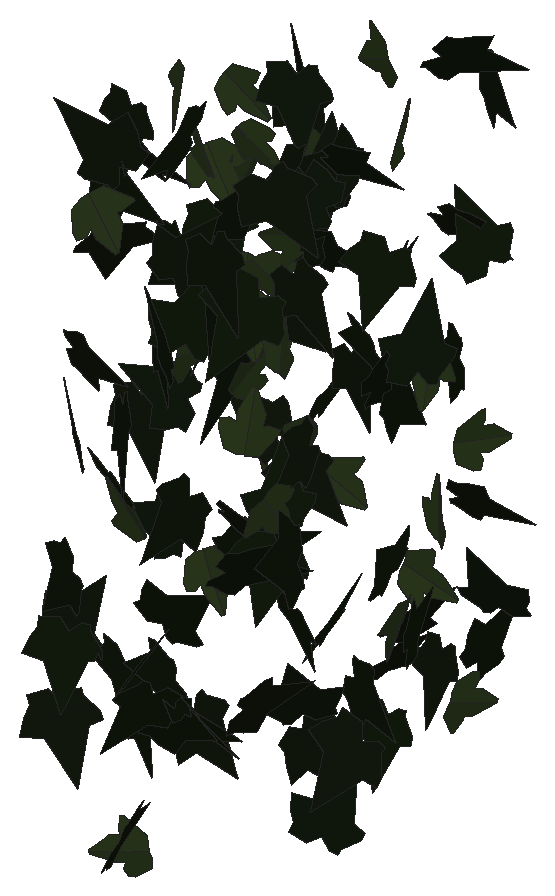
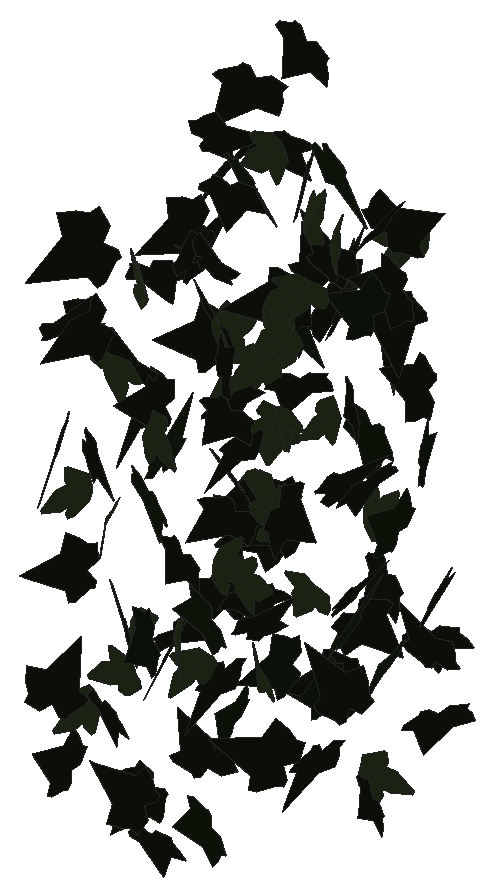
# SketchUp Ruby script. Lengths in inches.
U = 1.inch
M = Sketchup.active_model
def pt(a) = Geom::Point3d.new(a.map { |v| v * U })
def face(e, loops, mat)
  f = e.add_face(loops[0].map { |a| pt(a) })
  loops[1..].each { |l| e.add_face(l.map { |a| pt(a) }).erase! }
  f.material = f.back_material = mat if mat
  f
end
# faces: each face lists its corners as indices into pts; further lists are holes
def faces(e, pts, list, mat = nil) = list.each { |f| face(e, (f[0].is_a?(Array) ? f : [f]).map { |l| l.map { |i| pts[i] } }, mat) }
# xy, xz, yz: faces in a plane at the given z, y or x. An outline is a flat list of corners, or four numbers for a rectangle; further outlines are holes
def ring(l) = l.size == 4 ? [[l[0], l[1]], [l[2], l[1]], [l[2], l[3]], [l[0], l[3]]] : l.each_slice(2).to_a
def flat(e, list, mat, &to3) = list.each { |f| face(e, (f[0].is_a?(Array) ? f : [f]).map { |l| ring(l).map { |u, v| to3.(u, v) } }, mat) }
def xy(e, z, list, mat = nil) = flat(e, list, mat) { |x, y| [x, y, z] }
def xz(e, y, list, mat = nil) = flat(e, list, mat) { |x, z| [x, y, z] }
def yz(e, x, list, mat = nil) = flat(e, list, mat) { |y, z| [x, y, z] }
def lines(e, pts, list) = list.each { |a, b| e.add_line(pt(pts[a]), pt(pts[b])) }
# prism: a flat outline (further loops are holes) pulled along v
def prism(e, loops, v, mat = nil)
  f = face(e, loops, mat); d = Geom::Vector3d.new(v.map { |x| x * U })
  f.pushpull(f.normal.samedirection?(d) ? d.length : -d.length)
end
def box(e, o, s, mat = nil) = prism(e, [[o, [o[0] + s[0], o[1], o[2]], [o[0] + s[0], o[1] + s[1], o[2]], [o[0], o[1] + s[1], o[2]]]], [0, 0, s[2]], mat)
def at(x, y, z, deg = 0) = Geom::Transformation.translation(pt([x, y, z])) * Geom::Transformation.rotation(ORIGIN, Z_AXIS, deg.degrees)
def axes(o, x, y, z) = Geom::Transformation.new([*x, 0, *y, 0, *z, 0, *pt(o).to_a, 1])
def part(name) = M.definitions.add(name)
# library, detail: a bought-in or finely detailed component or shape, given as its bounding box
def library(name, o, s) = part(name).tap { |d| box(d.entities, o, s) }
def detail(e, o, s) = box(e.add_group.entities, o, s)
def put(e, d, t, mat = nil) = e.add_instance(d, t).tap { |i| i.material = mat if mat }
def group(e, t, mat = nil) = e.add_group.tap { |g| g.transformation = t; g.material = mat if mat }.entities
root = M.entities
M.materials.add("efeu1").color = [18, 25, 13]
M.materials.add("efeu2").color = [43, 57, 29]
c1 = part("ivyleaf_9")
p = [[1.54,2.16,1.25],[1.36,2.04,1.19],[-0.21,0.99,0.68],[-0.71,1.11,0.82],[-0.85,0.86,0.67],[-0.8,0.17,0.21],
  [-0.9,-0.01,0.1],[-0.67,-0.16,-0.02],[-0.08,-0.08,-0.05],[-0.03,-0.6,-0.4],[0.65,-0.88,-0.66],[0.83,-0.6,-0.49],
  [1.29,-0.42,-0.43],[1.8125,-0.07,-0.26],[1.21,0.44,0.15]]
faces(c1.entities,p,[[0,1,2,3,4,5,6,7,8,9,10,11,12,13,14]],"efeu1")
c2 = part("ivyleaf_10")
p = [[0,0.5,-0.03],[-0.0625,2.02,-0.43],[-0.19,2.01,-0.46],[-0.54,1.05,-0.29],[-0.52,0.625,-0.18],[-0.83,0.76,-0.28],
  [-1.16,0.64,-0.33],[-1.15,0.33,-0.24],[-0.77,-0.39,0.02],[-0.3,-0.51,0.16],[0.04,-0.48,0.23],[-0.02,2.01,-0.4375],
  [-0.06,2.01,-0.43],[0.04,-0.49,0.23],[0.67,-0.49,0.14],[1.38,0.36,-0.2],[1.375,0.51,-0.24],[0.81,0.65,-0.19],
  [0.62,0.59,-0.15],[0.6,1.09,-0.28],[0.5,1.23,-0.31]]
faces(c2.entities,p,[[0,1,2,3,4,5,6,7,8,9,10],[11,12,0,13,14,15,16,17,18,19,20]],"efeu2")
put(root,c1,axes([607.125,118.13,218.71],[-0.06969,-0.72711,1.04143],[-0.12365,-1.03416,-0.73031],[1.26411,-0.14124,-0.01402]))
put(root,c2,axes([608.34,131.87,225.82],[-0.15049,0.15579,-1.18714],[-1.04561,0.56581,0.20681],[0.58332,1.05442,0.06443]))
put(root,c1,axes([607.07,117.54,212.14],[-0.20534,-1.15684,-0.58674],[0.18534,0.56179,-1.1725],[1.28382,-0.26613,0.07542]))
put(root,c1,axes([607.15,117.79,215.54],[-0.72821,0.39761,0.96343],[0.84766,-0.45791,0.82968],[0.60644,1.1175,-0.00282]))
put(root,c1,axes([607.11,122.93,209.64],[-0.35959,-0.07566,-1.07282],[1.06754,0.11214,-0.36573],[0.13049,-1.12591,0.03566]))
put(root,c2,axes([607.3,131.73,220.83],[0.84987,-0.42418,0.82528],[0.73139,-0.38249,-0.94978],[0.57104,1.12119,-0.01179]))
put(root,c1,axes([606.91,123.26,238.16],[0.62383,-0.5405,0.88863],[0.78431,-0.43611,-0.81586],[0.68312,0.9943,0.12522]))
put(root,c1,axes([607.94,116.9,216.35],[-0.73327,-0.83517,-0.53296],[0.3557,0.39692,-1.11138],[0.92468,-0.81497,0.00488]))
put(root,c2,axes([609.09,138.31,237.18],[-0.51651,0.08232,1.14371],[-1.13111,0.16937,-0.52301],[-0.18826,-1.24345,0.00448]))
put(root,c1,axes([609.2,118.88,240.29],[0.01514,0.07865,1.42004],[-1.27605,0.62783,-0.02117],[-0.62801,-1.2738,0.07725]))
put(root,c1,axes([607.7,133.79,236.8],[-0.41526,-0.3402,-1.02342],[0.79143,0.64887,-0.53682],[0.73264,-0.89375,-0.00018]))
put(root,c1,axes([608.76,116.77,225.93],[0.08328,-0.59828,1.07913],[-0.19945,1.06084,0.60353],[-1.21766,-0.21468,-0.02505]))
put(root,c1,axes([607.24,120.49,238.24],[0.41428,-0.11876,-1.276],[1.18799,0.53849,0.33558],[0.48059,-1.22875,0.2704]))
put(root,c1,axes([607.46,129.98,214.55],[0.32547,-0.00545,1.28688],[1.27044,0.21297,-0.32041],[-0.20515,1.31021,0.05744]))
put(root,c2,axes([607.63,129.2,239.375],[0.63798,0.15904,0.93735],[0.84731,0.41693,-0.64743],[-0.43126,1.05443,0.11462]))
put(root,c1,axes([608.76,119.17,236.34],[0.34199,1.13401,-0.50168],[-0.16751,-0.47339,-1.18426],[-1.22866,0.38019,0.02182]))
put(root,c1,axes([608.23,121.09,241.83],[0.05618,-1.10787,0.34564],[0.00931,-0.34561,-1.10927],[1.1605,0.0564,-0.00783]))
put(root,c1,axes([608.95,138.74,225.16],[0.09159,0.5394,1.16111],[0.16037,1.15007,-0.54692],[-1.2702,0.18409,0.01467]))
put(root,c1,axes([609.52,129.83,221.62],[-0.64673,-0.95272,-0.09064],[-0.03111,-0.08841,1.15124],[-0.95651,0.64704,0.02384]))
put(root,c1,axes([609.41,132.28,237.67],[0.22896,-0.44574,1.13082],[-0.33111,1.08432,0.49446],[-1.16954,-0.39425,0.0814]))
put(root,c1,axes([608.1,119.67,223.49],[0.57206,-0.87365,0.76184],[0.51485,-0.56967,-1.03987],[1.03856,0.76363,0.09586]))
put(root,c1,axes([607.99,117.43,230.86],[0.5832,0.12374,-1.09187],[1.054,0.2866,0.59545],[0.31077,-1.20423,0.02952]))
put(root,c2,axes([608.54,124.2,242.01],[0.2695,-0.59009,1.02367],[0.74125,-0.73322,-0.61781],[0.92014,0.76349,0.19787]))
put(root,c1,axes([608.71,121.34,226.88],[0.12098,-1.28378,-0.24874],[-0.02323,0.24765,-1.28947],[1.30745,0.12319,0.00011]))
put(root,c1,axes([609.42,122.55,219.99],[0.13164,-1.06979,-0.31163],[0.04075,-0.30896,1.07786],[-1.11351,-0.13777,0.0026]))
put(root,c1,axes([609.83,122.94,226.63],[-0.37965,-1.06536,-0.4059],[-0.04871,-0.41227,1.12762],[-1.13902,0.37272,0.08707]))
put(root,c1,axes([608.67,123.02,214.5625],[-0.206,-0.17401,1.28979],[1.14404,-0.6468,0.09546],[0.6205,1.13475,0.25219]))
put(root,c1,axes([609.4,126.01,234.66],[-0.29536,-0.97904,-0.61849],[0.29625,0.55317,-1.01712],[1.1195,-0.40468,0.10598]))
put(root,c2,axes([610.375,134.77,222.94],[-0.07802,0.12604,-1.2232],[-0.58849,1.07236,0.14804],[1.07971,0.59359,-0.0077]))
put(root,c2,axes([609.45,116.96,238.98],[0.58533,0.96556,0.5108],[0.2424,0.45025,-1.12887],[-1.06511,0.63309,0.0238]))
put(root,c1,axes([609.18,127.04,218.49],[1.09469,-0.34863,0.37768],[0.36731,-0.09101,-1.14863],[0.35955,1.15443,0.02351]))
put(root,c1,axes([609.49,119.08,214.35],[0.28261,-1.21211,0.68621],[0.17416,-0.66395,-1.24452],[1.38195,0.33156,0.01651]))
put(root,c1,axes([610.12,126.54,227.13],[-0.34444,0.40732,-1.32647],[0.85397,-1.01502,-0.53343],[-1.0937,-0.92081,0.00124]))
put(root,c2,axes([610.89,118.05,222.45],[-0.90035,0.47876,-0.7305],[-0.70109,0.22951,1.01452],[0.52087,1.13648,0.10285]))
put(root,c1,axes([610.64,131.84,210.52],[-0.68328,0.9741,-0.54665],[-0.31471,0.44698,1.18985],[1.07175,0.75227,0.00087]))
put(root,c2,axes([610.3,131.625,235.52],[-0.13307,0.26768,1.12161],[0.39601,-1.04978,0.29752],[1.08298,0.41676,0.02903]))
put(root,c1,axes([610.77,131.62,222.6],[-0.69132,1.03275,-0.38791],[-0.21567,0.32243,1.24278],[1.08191,0.72418,-0.00013]))
put(root,c1,axes([610.0625,120.79,230.77],[-0.227,-0.02944,-1.14512],[1.13995,-0.12054,-0.22287],[-0.11259,-1.16116,0.05217]))
put(root,c2,axes([610.6,126.24,226.15],[0.17923,-0.84537,0.85057],[-0.07833,0.84993,0.86124],[-1.19666,-0.18225,0.07102]))
put(root,c2,axes([610.66,126.17,232.32],[1.16699,-0.02123,-0.01332],[-0.01328,0.0022,-1.16718],[0.02125,1.16707,0.00196]))
put(root,c2,axes([610.5,124.05,238.8],[0.91558,0.61837,0.57447],[0.48038,0.31512,-1.10482],[-0.694,1.03392,-0.00686]))
put(root,c1,axes([610.8125,122.53,210.74],[0.38874,-0.82439,-0.94465],[-0.31801,0.89184,-0.90918],[1.21279,0.4981,0.06439]))
put(root,c2,axes([611.08,121.34,230.05],[-0.12838,-0.3064,-1.08654],[0.31439,1.04058,-0.33058],[1.08425,-0.33801,-0.03279]))
put(root,c2,axes([612.08,116.81,206.68],[-0.23295,-0.03972,1.18082],[-1.05668,-0.5314,-0.22633],[0.52853,-1.07992,0.06795]))
put(root,c2,axes([611.22,125.95,238.08],[0.21181,-0.81862,0.86179],[0.23565,-0.82907,-0.84546],[1.16503,0.31653,0.01433]))
put(root,c1,axes([611.1,120.93,235.32],[-0.10319,-0.57856,1.09148],[-0.15111,-1.08114,-0.58737],[1.22606,-0.18194,0.01948]))
put(root,c1,axes([611.0625,129.66,234.52],[-0.22423,-1.13381,-0.17658],[0.0278,0.1745,-1.15575],[1.14714,-0.22585,-0.00651]))
put(root,c2,axes([611.5,125.34,230.79],[0.93898,0.73102,0.25634],[0.20847,0.1495,-1.18995],[-0.74609,0.9618,-0.00987]))
put(root,c2,axes([611.77,131.15,219.55],[0.3516,0.76088,0.81894],[0.25202,0.78243,-0.83517],[-1.08907,0.42671,0.07112]))
put(root,c2,axes([612.63,121.04,240.53],[-0.88135,0.69312,-0.54075],[-0.42078,0.3397,1.12123],[0.77186,0.97662,-0.00622]))
put(root,c1,axes([612.2,126.8125,230.53],[0.3844,-0.55002,-1.00228],[-0.3336,0.95744,-0.65335],[1.09353,0.48543,0.15301]))
put(root,c1,axes([613.4,118.79,243.16],[-1.04847,0.98431,-0.03793],[0.02616,-0.02755,-1.4381],[-0.98469,-1.04879,0.00218]))
put(root,c1,axes([612.66,118.56,214.93],[0.70046,-1.19278,-0.39127],[0.21424,-0.32789,1.38313],[-1.2369,-0.73227,0.01799]))
put(root,c2,axes([612.13,121.59,219.46],[0.99241,0.15588,0.66927],[0.6589,0.11796,-1.00451],[-0.19512,1.19117,0.0119]))
put(root,c2,axes([612.79,128.02,223.54],[0.0644,-0.72297,0.95503],[0.16634,-0.94174,-0.72413],[1.18621,0.17131,0.0497]))
put(root,c1,axes([612.28,122.91,237.03],[0.12149,0.78523,-1.06368],[0.09415,1.06031,0.7935],[1.31876,-0.14804,0.04134]))
put(root,c1,axes([613.22,116.31,215.26],[-0.06615,0.49094,-1.10293],[0.05956,-1.10191,-0.49406],[-1.20579,-0.08136,0.0361]))
put(root,c1,axes([612.08,118.51,212.86],[0.23665,0.37007,-1.21995],[0.69547,1.00242,0.43899],[1.06844,-0.73446,-0.01554]))
put(root,c1,axes([612.33,127.74,214.32],[0.48659,-0.93384,0.64277],[0.29429,-0.57145,-1.05301],[1.09481,0.56866,-0.00263]))
put(root,c1,axes([612.5625,131.67,225.8],[-0.51045,-0.18358,-1.04783],[0.99918,0.31614,-0.54214],[0.3651,-1.12186,0.01869]))
put(root,c1,axes([613.09,140.67,236.8],[0.82561,-0.46307,-1.0576],[-0.92622,0.51055,-0.94659],[0.68925,1.24076,-0.00521]))
put(root,c1,axes([612.42,119.77,212.74],[0.87208,-0.52992,0.60038],[0.52753,-0.28767,-1.02017],[0.60249,1.01893,0.02422]))
put(root,c2,axes([613.06,124.52,233.82],[-0.93165,-0.32143,-0.71865],[0.68813,0.2084,-0.98529],[0.38243,-1.15802,0.02216]))
put(root,c1,axes([612.87,114.68,230.6],[-0.49511,0.02108,-1.37483],[1.35377,-0.24824,-0.49134],[-0.24062,-1.44002,0.06457]))
put(root,c1,axes([613.19,118.13,236.27],[-0.65597,0.41545,1.05394],[0.89118,-0.56266,0.77646],[0.69942,1.10657,-0.00088]))
put(root,c1,axes([614,124.4,219.72],[-0.71173,-1.02965,-0.22299],[0.13251,0.17947,-1.25168],[1.04516,-0.72393,0.00685]))
put(root,c1,axes([614.29,120.42,234.27],[-0.87808,0.55744,-0.80683],[0.65722,-0.4693,-1.0395],[-0.72786,-1.09625,0.03474]))
put(root,c2,axes([614.46,125.69,235.47],[-0.25932,-0.31325,-1.17019],[-0.55034,-1.03561,0.39918],[-1.07917,0.6034,0.07762]))
put(root,c1,axes([613.86,133.32,211.44],[0.48214,1.1165,-0.16894],[0.0308,0.17062,1.21553],[1.12878,-0.48155,0.03899]))
put(root,c1,axes([614.52,125.23,243.79],[-0.77278,-0.62348,-0.78307],[0.57645,0.53156,-0.9921],[0.81831,-0.96324,-0.04062]))
put(root,c1,axes([615.1875,115.11,233.79],[0.25403,-0.96814,0.77944],[-0.0517,0.78663,0.99392],[-1.24183,-0.23079,0.11807]))
put(root,c1,axes([614.88,131.39,211.16],[0.50625,0.90453,0.56899],[0.23313,0.52096,-1.0356],[-1.04287,0.55556,0.04471]))
put(root,c1,axes([614.94,131.16,208.25],[-0.92146,-0.42365,-0.59746],[0.54207,0.25125,-1.01418],[0.49255,-1.06907,-0.00159]))
put(root,c1,axes([614.7,125.57,234.94],[-0.51283,0.714,0.85246],[0.49797,-0.69189,0.87909],[0.99423,0.71482,-0.00059]))
put(root,c1,axes([615.22,116.36,234.38],[-1.00961,0.02098,0.93039],[0.92421,-0.13827,1.00603],[0.10906,1.36595,0.08755]))
put(root,c1,axes([615.98,122.34,223],[-1.13322,-0.05731,0.31312],[0.31325,0.00496,1.13462],[-0.05656,1.17567,0.01048]))
put(root,c1,axes([614.99,124.42,224.25],[-0.07423,-0.43959,-1.14988],[0.66698,0.95388,-0.40772],[1.0347,-0.64641,0.18033]))
put(root,c1,axes([614.93,125.8,234.95],[0.88458,-0.1317,0.83067],[0.82475,-0.1003,-0.89418],[0.16474,1.20931,0.0163]))
put(root,c1,axes([616.22,125.12,238.5],[-1.20902,0.19968,0.29566],[0.28979,-0.0597,1.22534],[0.2081,1.24321,0.01135]))
put(root,c1,axes([616.52,123.45,226.17],[-1.20746,0.29739,-0.32961],[0.3216,-0.07253,-1.24352],[-0.30604,-1.24953,-0.00626]))
put(root,c2,axes([616.15,121.09,224.12],[-0.28329,-0.99616,-0.6593],[0.29696,0.59759,-1.03051],[1.15707,-0.39726,0.10306]))
put(root,c2,axes([615.63,120.31,243.38],[-0.72563,0.15262,-0.89165],[0.87597,-0.16683,-0.74143],[-0.22584,-1.13743,-0.0109]))
put(root,c1,axes([615.74,118.81,221.47],[0.93321,0.66225,0.92681],[0.69661,0.61617,-1.14171],[-0.90127,1.16198,0.07721]))
put(root,c1,axes([616.55,126.12,238.89],[-0.14719,0.10415,1.38679],[-0.72917,-1.19326,0.01223],[1.18421,-0.72179,0.17989]))
put(root,c1,axes([616.15,128.7,228.68],[0.91098,-1.00075,-0.24613],[0.16705,-0.18077,1.35328],[-1.01694,-0.92617,0.00182]))
put(root,c2,axes([616.78,129.64,238.92],[0.76405,-0.98172,0.0503],[-0.0291,0.04109,1.244],[-0.98258,-0.7646,0.00227]))
put(root,c1,axes([617.77,120.58,241.86],[-0.96219,0.81642,0.17396],[-0.13766,0.10664,-1.26186],[-0.82332,-0.97196,0.00768]))
put(root,c1,axes([617.57,108.6875,212.71],[-0.52187,0.51634,-1.11801],[-0.77819,0.80283,0.73403],[0.95445,0.93689,-0.01283]))
put(root,c2,axes([617.6875,119.93,232.64],[-0.05126,0.89413,-0.80109],[-0.15925,0.78966,0.89157],[1.18989,0.14421,0.08481]))
put(root,c2,axes([617.39,117.91,229.26],[0.57238,0.98736,-0.39768],[0.19486,0.34671,1.14125],[1.04645,-0.60462,0.005]))
put(root,c1,axes([618.06,109.33,221.48],[-0.19943,1.20599,0.54151],[-0.10581,0.53131,-1.22226],[-1.31774,-0.22518,0.01619]))
put(root,c1,axes([616.87,124.9,240.59],[1.10311,0.22395,0.4935],[0.47968,0.11736,-1.12547],[-0.2522,1.20275,0.01793]))
put(root,c2,axes([616.98,130.56,216.77],[0.32173,0.17186,1.13073],[1.05521,0.40847,-0.36233],[-0.44115,1.10237,-0.04203]))
put(root,c1,axes([617.3125,132.46,242.72],[1.07147,0.65684,0.75711],[0.6213,0.43444,-1.25617],[-0.78654,1.23795,0.03912]))
put(root,c1,axes([617.82,121.67,212.7],[0.43731,-0.7398,-1.03712],[-0.45684,0.93253,-0.85782],[1.18921,0.63028,0.05185]))
put(root,c1,axes([617.89,114.94,238.3],[0.39119,-0.26758,-1.36632],[1.22833,-0.60184,0.46954],[-0.65548,-1.2875,0.06448]))
put(root,c1,axes([618.35,122.34,207.34],[-0.77616,-0.0401,1.00768],[0.99503,-0.23741,0.75697],[0.16414,1.24959,0.17616]))
put(root,c1,axes([618.67,133.21,211.75],[-0.08063,-0.10995,1.24239],[0.69187,1.03194,0.13623],[-1.03776,0.69653,-0.00571]))
put(root,c1,axes([619.81,130.21,228.96],[-0.12632,0.01454,-1.19902],[-1.19884,-0.02682,0.12597],[-0.02515,1.20535,0.01727]))
put(root,c2,axes([619.17,126.96,217.12],[0.3397,-1.19723,0.22203],[0.06448,-0.2125,-1.24448],[1.21593,0.34574,0.00396]))
put(root,c1,axes([619.03,111.68,229.53],[0.14443,-0.16201,-1.36442],[0.68449,-1.18109,0.2127],[-1.19136,-0.69823,-0.04321]))
put(root,c1,axes([619.04,125.12,229.32],[0.26414,0.18887,1.19966],[0.65099,1.0144,-0.30304],[-1.02522,0.69279,0.11666]))
put(root,c1,axes([619.27,129.7,213.76],[-0.93864,-0.0812,-0.74508],[0.74121,0.07648,-0.94209],[0.11113,-1.19597,-0.00965]))
put(root,c1,axes([619.36,119.625,215.17],[0.88852,0.37828,0.81149],[-0.74655,-0.31809,0.96569],[0.49424,-1.16052,-0.00018]))
put(root,c1,axes([619.39,123.41,215.125],[0.82762,-0.64744,-0.86758],[-0.63438,0.59484,-1.04907],[0.87718,1.04106,0.05987]))
put(root,c1,axes([620.72,119.33,241.94],[-0.49827,0.04659,1.06697],[-1.06501,0.06613,-0.50025],[-0.07965,-1.17572,0.01414]))
put(root,c1,axes([619.98,132.88,215.15],[0.93382,-0.21529,0.81178],[-0.79027,0.18568,0.95831],[-0.28428,-1.22333,0.00259]))
put(root,c1,axes([619.9375,125.4,229.41],[0.42549,-0.30275,-1.14645],[-0.82027,0.8044,-0.51686],[0.85624,0.92105,0.07455]))
put(root,c1,axes([619.35,130.07,236.17],[1.21712,0.15965,0.26245],[0.26032,0.03331,-1.22755],[-0.16309,1.24465,-0.00081]))
put(root,c1,axes([619.84,114.95,217.54],[-0.09215,0.79079,-1.01641],[-0.19547,0.99861,0.79466],[1.27288,0.2106,0.04845]))
put(root,c1,axes([619.84,126.68,215.69],[-0.35522,0.88898,0.8258],[0.16693,-0.81648,0.95075],[1.20182,0.37616,0.11202]))
put(root,c1,axes([620.16,124.7,236.83],[-0.8625,-0.80279,-0.27239],[0.19801,0.18706,-1.17829],[0.8243,-0.88493,-0.00197]))
put(root,c1,axes([620.12,116.3,244.2],[-0.31349,-0.55199,-1.21016],[0.59267,1.05511,-0.63479],[1.19077,-0.67047,-0.00265]))
put(root,c1,axes([620.98,114.23,239.37],[-1.1995,-0.83443,-0.04972],[0.04938,0.01608,-1.46111],[0.83445,-1.20042,0.01499]))
put(root,c1,axes([619.94,130.38,221.74],[0.9574,-0.11575,0.72856],[0.73128,-0.00818,-0.96228],[0.09709,1.20306,0.06355]))
put(root,c2,axes([621.34,126.75,222.27],[-0.13046,0.74801,-1.01828],[-0.36691,0.95715,0.75012],[1.20905,0.37118,0.11776]))
put(root,c1,axes([621.29,125.53,231.05],[-1.29816,0.31772,0.36336],[0.35148,-0.09235,1.33646],[0.33082,1.34489,0.00593]))
put(root,c1,axes([621.59,130.11,234.89],[-0.88029,-0.80384,0.22475],[0.17253,0.14435,1.19204],[-0.81664,0.89699,0.00957]))
put(root,c1,axes([621.07,116.89,224.66],[-0.18615,-0.2685,1.46453],[-0.31587,-1.43522,-0.30327],[1.45505,-0.34591,0.12152]))
put(root,c2,axes([621.09,129.27,225.48],[0.07007,0.14711,1.19445],[0.08129,1.19316,-0.15172],[-1.20073,0.08937,0.05943]))
put(root,c1,axes([622.0625,122.53,222.07],[-0.36986,0.93071,0.81343],[-0.31763,0.74899,-1.0014],[-1.19457,-0.48731,0.01441]))
put(root,c1,axes([621.43,121.08,213.65],[-0.65595,-1.11147,0.48067],[-0.22288,-0.42651,-1.29038],[1.19026,-0.69239,0.02327]))
put(root,c2,axes([621.32,128.375,212.59],[-0.18348,-0.43758,-1.10288],[0.43783,1.01226,-0.47446],[1.10278,-0.4747,0.00488]))
put(root,c2,axes([621.43,126.07,231.46],[1.26113,-0.01434,0.0856],[0.08569,0.00762,-1.26119],[0.01379,1.26401,0.00857]))
put(root,c1,axes([621.12,116.875,239.4375],[0.6093,-1.12139,-0.48044],[-0.15467,0.46169,-1.27378],[1.21013,0.62363,0.0791]))
put(root,c1,axes([621.21,110.77,243.61],[-0.60299,-0.24379,-1.24831],[1.14783,0.49083,-0.6503],[0.54792,-1.29652,-0.01146]))
